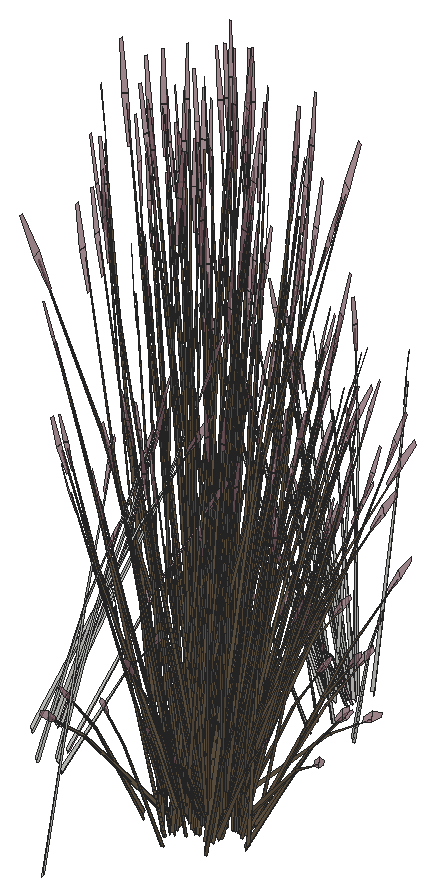
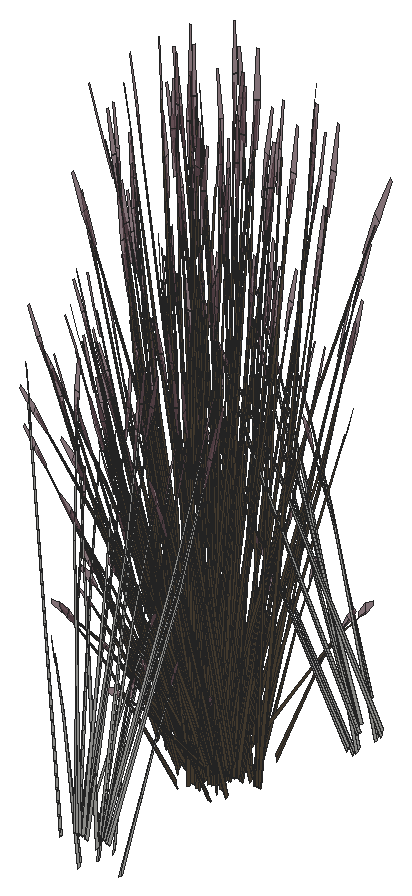
# SketchUp Ruby script. Lengths in inches.
U = 1.inch
M = Sketchup.active_model
def pt(a) = Geom::Point3d.new(a.map { |v| v * U })
def face(e, loops, mat)
  f = e.add_face(loops[0].map { |a| pt(a) })
  loops[1..].each { |l| e.add_face(l.map { |a| pt(a) }).erase! }
  f.material = f.back_material = mat if mat
  f
end
# faces: each face lists its corners as indices into pts; further lists are holes
def faces(e, pts, list, mat = nil) = list.each { |f| face(e, (f[0].is_a?(Array) ? f : [f]).map { |l| l.map { |i| pts[i] } }, mat) }
# xy, xz, yz: faces in a plane at the given z, y or x. An outline is a flat list of corners, or four numbers for a rectangle; further outlines are holes
def ring(l) = l.size == 4 ? [[l[0], l[1]], [l[2], l[1]], [l[2], l[3]], [l[0], l[3]]] : l.each_slice(2).to_a
def flat(e, list, mat, &to3) = list.each { |f| face(e, (f[0].is_a?(Array) ? f : [f]).map { |l| ring(l).map { |u, v| to3.(u, v) } }, mat) }
def xy(e, z, list, mat = nil) = flat(e, list, mat) { |x, y| [x, y, z] }
def xz(e, y, list, mat = nil) = flat(e, list, mat) { |x, z| [x, y, z] }
def yz(e, x, list, mat = nil) = flat(e, list, mat) { |y, z| [x, y, z] }
def lines(e, pts, list) = list.each { |a, b| e.add_line(pt(pts[a]), pt(pts[b])) }
# prism: a flat outline (further loops are holes) pulled along v
def prism(e, loops, v, mat = nil)
  f = face(e, loops, mat); d = Geom::Vector3d.new(v.map { |x| x * U })
  f.pushpull(f.normal.samedirection?(d) ? d.length : -d.length)
end
def box(e, o, s, mat = nil) = prism(e, [[o, [o[0] + s[0], o[1], o[2]], [o[0] + s[0], o[1] + s[1], o[2]], [o[0], o[1] + s[1], o[2]]]], [0, 0, s[2]], mat)
def at(x, y, z, deg = 0) = Geom::Transformation.translation(pt([x, y, z])) * Geom::Transformation.rotation(ORIGIN, Z_AXIS, deg.degrees)
def axes(o, x, y, z) = Geom::Transformation.new([*x, 0, *y, 0, *z, 0, *pt(o).to_a, 1])
def part(name) = M.definitions.add(name)
# library, detail: a bought-in or finely detailed component or shape, given as its bounding box
def library(name, o, s) = part(name).tap { |d| box(d.entities, o, s) }
def detail(e, o, s) = box(e.add_group.entities, o, s)
def put(e, d, t, mat = nil) = e.add_instance(d, t).tap { |i| i.material = mat if mat }
def group(e, t, mat = nil) = e.add_group.tap { |g| g.transformation = t; g.material = mat if mat }.entities
root = M.entities
M.materials.add("Forest_Floor_01_1K").color = [106, 91, 72]
M.materials.add("LightPink_Translucent").color = [144, 107, 117]
M.materials["LightPink_Translucent"].alpha = 0.75
c1 = part("blade")
p = [[2.15,0.21,22],[0,0.17,0],[0.09,0.45,0],[2.18,0.31,22],[2.29,0.31,22],[0.38,0.45,0],
  [2.48,0.24,33],[2.49,0.24,33],[2.48,0.22,33]]
faces(c1.entities,p,[[0,1,2,3],[4,5,2,3],[6,3,4,7],[8,0,3,6]])
c2 = part("seeds")
p = [[0.3,-0.1,1.38],[-0.01,-0.03,1.59],[-0.01,-0.03,0.03],[0.14,-0.07,-0.07],[0.29,-0.03,3],[0.15,0.01,3.11]]
faces(c2.entities,p,[[0,1,2,3],[1,0,4,5]],"LightPink_Translucent")
c3 = part("blade with seeds")
put(c3.entities,c1,at(0,0,0))
put(c3.entities,c2,axes([2.4,0.25,30.99],[1.5799,-0.05474,1.17369],[-0.12525,1.92788,0.29478],[-0.07173,-0.02425,1.56792]))
put(root,c3,axes([508.54,142.77,4.23],[-0.74352,0.28449,-0.1216],[-0.36538,-0.50492,-0.67495],[-0.0981,-0.21277,1.02557]))
put(root,c3,axes([507.23,125.56,1.52],[-0.70674,0.51372,0.30756],[-0.70717,-0.50832,-0.36492],[-0.02468,-0.14589,1.64885]),"Forest_Floor_01_1K")
put(root,c3,axes([507.9,142.8,3.875],[-0.7469,-0.15318,-0.51099],[0.25601,-0.52518,-0.3958],[-0.06849,-0.21144,0.97773]))
put(root,c3,axes([500.09,120.04,5.39],[-0.27143,-0.0181,1.43002],[-0.27808,-0.48551,-0.30754],[0.33346,-0.13735,0.61141]))
put(root,c3,axes([510.14,126.98,2.52],[0.65659,0.2464,1.51261],[-0.64324,0.53082,0.59816],[-0.28812,-0.31461,1.26806]),"Forest_Floor_01_1K")
put(root,c3,axes([500.28,121.75,7.33],[0.63144,0.17046,-0.35414],[-0.18417,0.49731,0.4572],[0.25423,-0.0456,0.87481]))
put(root,c3,axes([507.64,122.51,1.96],[0.39634,0.21267,1.1486],[-0.57721,0.12784,0.84392],[-0.1235,-0.16344,0.25299]),"Forest_Floor_01_1K")
put(root,c3,axes([510.43,126.81,1.66],[-0.74193,-0.49181,-0.25192],[0.6243,-0.55226,0.5513],[-0.19979,0.05753,1.68216]),"Forest_Floor_01_1K")
put(root,c3,axes([509.08,126.33,1.4],[-0.45644,-0.51287,-0.44739],[0.69137,-0.36116,0.21531],[-0.14771,-0.06346,1.43643]),"Forest_Floor_01_1K")
put(root,c3,axes([499.06,122.82,7.78],[0.75952,0.01471,-0.71045],[-0.05101,0.61953,0.08574],[0.32177,0.06538,1.00501]))
put(root,c3,axes([507.79,127.6875,4.53],[-0.01977,0.56521,-0.7886],[-0.83252,-0.03796,0.09517],[-0.08786,0.23945,1.11556]),"Forest_Floor_01_1K")
put(root,c3,axes([500.6,121.65,4.78],[-0.48937,0.07333,1.41583],[-0.07789,-0.58369,0.08104],[0.34275,-0.08835,0.80566]))
put(root,c3,axes([507.77,129.28,1.96],[-0.01966,-0.36332,1.1486],[0.49135,0.25914,0.84392],[-0.09663,0.17317,0.25299]),"Forest_Floor_01_1K")
put(root,c3,axes([508.46,123.07,4.29],[0.84639,-0.15705,0.53763],[0.14689,0.61608,0.4433],[-0.19906,-0.18157,1.11249]),"Forest_Floor_01_1K")
put(root,c3,axes([501.13,121.27,4.29],[-0.03971,-0.09277,1.76342],[0.27541,-0.54264,-0.26939],[0.27782,-0.00781,0.30037]))
put(root,c3,axes([510.05,126.7,1.4],[-0.82508,0.03772,-0.44739],[-0.07462,-0.62614,0.21531],[-0.14771,0.06346,1.43643]),"Forest_Floor_01_1K")
put(root,c3,axes([508.17,142.9,4.17],[-0.36264,-0.49684,-0.71045],[0.74649,-0.27689,0.08574],[-0.0848,-0.24006,1.00501]))
put(root,c3,axes([498.56,121.14,6.68],[-0.31515,0.01384,1.71376],[0.20907,-0.5998,0.13857],[0.44912,0.0371,0.73262]))
put(root,c3,axes([508.66,123.2,3.92],[0.34533,-0.38816,0.0643],[0.49176,0.22599,0.50621],[-0.15898,-0.12445,0.77189]),"Forest_Floor_01_1K")
put(root,c3,axes([507.4,110.87,2.56],[0.01669,-0.31544,1.54345],[0.75083,0.16661,0.21329],[-0.06506,0.33618,0.72882]))
put(root,c3,axes([508.48,127.75,1.67],[0.7111,0.30552,0.49651],[-0.42504,0.54784,0],[-0.16196,-0.06958,1.57504]),"Forest_Floor_01_1K")
put(root,c3,axes([507.51,128.49,2.56],[0.01669,-0.31544,1.54345],[0.75083,0.16661,0.21329],[-0.06506,0.33618,0.72882]),"Forest_Floor_01_1K")
put(root,c3,axes([499.71,121.7,7.78],[0.66765,-0.26986,-0.71045],[0.37208,0.55551,0.08574],[0.32259,-0.0631,1.00501]))
put(root,c3,axes([509.15,126.63,1.63],[0.20138,-0.72405,-0.23429],[0.95485,0.12621,0.51271],[-0.16685,-0.09999,1.5644]),"Forest_Floor_01_1K")
put(root,c3,axes([508.32,142.97,4.24],[-0.22906,0.4699,0.35414],[-0.66828,-0.13705,-0.4572],[-0.06128,-0.18919,0.87481]))
put(root,c3,axes([509.5,126.8,1.81],[-0.14658,0.54532,0.1448],[-0.71613,-0.09466,-0.41347],[-0.13033,-0.05599,1.26744]),"Forest_Floor_01_1K")
put(root,c3,axes([509.41,122.05,3.91],[-0.11621,-0.08567,1.74944],[-0.77555,0.05431,-0.27667],[-0.12378,-0.20491,0.14031]),"Forest_Floor_01_1K")
put(root,c3,axes([510.92,128.32,1.21],[-0.7111,0.30552,-0.49651],[-0.42504,-0.54784,0],[-0.16196,0.06958,1.57504]),"Forest_Floor_01_1K")
put(root,c3,axes([506.71,125.27,1.21],[0,-0.61104,-0.49651],[0.85008,0,0],[0,-0.13917,1.57504]),"Forest_Floor_01_1K")
put(root,c3,axes([507.08,125.84,1.67],[0,0.61104,0.49651],[-0.85008,0,0],[0,-0.13917,1.57504]),"Forest_Floor_01_1K")
put(root,c3,axes([510.97,128.16,1.39],[-0.46912,-0.61443,-0.05142],[0.79476,-0.34146,0.51607],[-0.19584,0.0585,1.6363]),"Forest_Floor_01_1K")
put(root,c3,axes([507.96,127.875,4.2],[0.54391,0.41056,-0.5672],[-0.57458,0.35956,-0.43934],[-0.08276,0.2086,1.08528]),"Forest_Floor_01_1K")
put(root,c3,axes([510.75,128.08,1.22],[-0.70886,-0.15119,-0.30978],[0.17848,-0.53243,0.30978],[-0.1429,0.0614,1.38974]),"Forest_Floor_01_1K")
put(root,c3,axes([507.72,127.57,4.24],[0.5141,-0.32171,0.35414],[0.48666,0.36734,-0.4572],[-0.07405,0.18664,0.87481]),"Forest_Floor_01_1K")
put(root,c3,axes([500.74,122.52,5.39],[-0.18299,-0.15028,1.43002],[0.23809,-0.49714,-0.30754],[0.37023,0.06735,0.61141]))
put(root,c3,axes([508.93,125.98,1.86],[-0.85568,-0.29155,-0.29095],[0.41201,-0.61537,-0.50002],[-0.02689,-0.15109,1.59708]),"Forest_Floor_01_1K")
put(root,c3,axes([511.16,125.8,2.03],[-0.02076,-0.57531,1.41272],[0.93937,0.14913,0.59816],[-0.22217,0.31481,1.3335]),"Forest_Floor_01_1K")
put(root,c3,axes([507.55,141.8,0.6875],[-0.12744,0.02202,1.76342],[-0.70477,-0.24781,-0.26939],[0.01183,-0.2067,0.30037]))
put(root,c3,axes([507.39,127.66,4.59],[0.83505,0.03027,-0.13498],[-0.02282,0.57322,-0.74919],[-0.05801,0.22077,1.13838]),"Forest_Floor_01_1K")
put(root,c3,axes([508.24,142.48,3.72],[0.22906,-0.4699,-0.35414],[0.66828,0.13705,0.4572],[-0.06128,-0.18919,0.87481]))
put(root,c3,axes([507.37,128.49,2.02],[0.69024,-0.1082,0.06507],[0.15868,0.43593,-0.86304],[-0.04376,0.22067,0.7736]),"Forest_Floor_01_1K")
put(root,c3,axes([510.63,126.53,1.86],[0.08854,0.69723,-0.29095],[-0.92215,0.04216,-0.50002],[-0.16238,0.09287,1.59708]),"Forest_Floor_01_1K")
put(root,c3,axes([508.55,125.36,1.29],[-0.31203,-0.62659,-0.69835],[0.89884,-0.22566,-0.18329],[-0.03449,-0.21218,1.54149]),"Forest_Floor_01_1K")
put(root,c3,axes([510.59,123.37,4.23],[-0.74352,0.28449,-0.1216],[-0.36538,-0.50492,-0.67495],[-0.0981,-0.21277,1.02557]),"Forest_Floor_01_1K")
put(root,c3,axes([509.96,123.4,3.875],[-0.7469,-0.15318,-0.51099],[0.25601,-0.52518,-0.3958],[-0.06849,-0.21144,0.97773]),"Forest_Floor_01_1K")
put(root,c3,axes([508.58,127.29,3.07],[-0.0186,-0.23452,1.71376],[0.80601,0.15558,0.13857],[-0.04985,0.33422,0.73262]),"Forest_Floor_01_1K")
put(root,c3,axes([507.08,125.29,1.22],[0.53038,-0.38124,-0.30978],[0.53038,0.38124,0.30978],[0,-0.1228,1.38974]),"Forest_Floor_01_1K")
put(root,c3,axes([509.47,122.82,1.32],[-0.52505,0.35054,-0.03893],[-0.48109,-0.38392,-0.17649],[-0.03387,-0.10878,0.58215]),"Forest_Floor_01_1K")
put(root,c3,axes([509.26,126.28,1.55],[0.96033,0.12874,0.45755],[-0.19544,0.7271,0.17955],[-0.14034,-0.07021,1.58856]),"Forest_Floor_01_1K")
put(root,c3,axes([509.01,126.15,1.91],[-0.36864,0.55059,0.44739],[-0.76598,-0.26498,-0.21531],[0,-0.12692,1.43643]),"Forest_Floor_01_1K")
put(root,c3,axes([510.23,123.5,4.17],[-0.36264,-0.49684,-0.71045],[0.74649,-0.27689,0.08574],[-0.0848,-0.24006,1.00501]),"Forest_Floor_01_1K")
put(root,c3,axes([508.52,142.54,3.92],[0.55987,-0.20767,0.0643],[0.27403,0.37869,0.50621],[-0.05407,-0.16693,0.77189]))
put(root,c3,axes([508.33,142.58,3.93],[0.74868,0.15974,0.48003],[-0.25601,0.52518,0.3958],[-0.04499,-0.20653,0.9933]))
put(root,c3,axes([508.74,127.44,1.67],[0.81646,-0.16218,0.17642],[0.20161,0.60355,0.35086],[-0.07282,-0.08794,1.60407]),"Forest_Floor_01_1K")
put(root,c3,axes([509.79,127.54,1.39],[-0.76598,-0.27433,0],[0.36864,-0.57001,0],[0,0,1.62707]),"Forest_Floor_01_1K")
put(root,c3,axes([510.37,123.57,4.24],[-0.22906,0.4699,0.35414],[-0.66828,-0.13705,-0.4572],[-0.06128,-0.18919,0.87481]),"Forest_Floor_01_1K")
put(root,c3,axes([511.57,128.22,1.57],[0.47504,0.61229,0],[-0.79476,0.34146,-0.51607],[-0.18101,0.07777,1.63711]),"Forest_Floor_01_1K")
put(root,c3,axes([509.15,128.49,4.26],[-0.74868,-0.15974,0.53283],[0.25601,-0.52518,0.43934],[0.04499,0.20653,1.10256]),"Forest_Floor_01_1K")
put(root,c3,axes([508.95,128.53,3.92],[-0.55987,0.20767,0.0643],[-0.27403,-0.37869,0.50621],[0.05407,0.16693,0.77189]),"Forest_Floor_01_1K")
put(root,c3,axes([511.17,127.47,1.67],[0.21949,-0.60727,0.17642],[0.8032,0.17185,0.35086],[-0.13875,0.00296,1.60407]),"Forest_Floor_01_1K")
put(root,c3,axes([510.8,126.67,1.81],[0.56134,0.36712,0.1448],[-0.46823,0.41419,-0.41347],[-0.13033,0.05599,1.26744]),"Forest_Floor_01_1K")
put(root,c3,axes([510.6,126.22,1.49],[-0.70674,-0.52593,-0.06131],[0.70717,-0.52625,0],[-0.02468,-0.01837,1.75571]),"Forest_Floor_01_1K")
put(root,c3,axes([510.79,126.4,1.91],[0.82508,-0.03772,0.44739],[0.07462,0.62614,-0.21531],[-0.14771,0.06346,1.43643]),"Forest_Floor_01_1K")
put(root,c3,axes([508.36,141.48,1.96],[0.09747,0.35631,1.1486],[-0.54071,-0.19735,0.84392],[0.05818,-0.18244,0.25299]))
put(root,c3,axes([510.99,127.84,1.52],[0.95122,0.19861,0.30756],[-0.23797,0.7099,-0.36492],[-0.15744,0.08885,1.64885]),"Forest_Floor_01_1K")
put(root,c3,axes([509.6,122.39,0.6875],[-0.12744,0.02202,1.76342],[-0.70477,-0.24781,-0.26939],[0.01183,-0.2067,0.30037]),"Forest_Floor_01_1K")
put(root,c3,axes([511.4,127.8,1.67],[0.7111,-0.30552,0.49651],[0.42504,0.54784,0],[-0.16196,0.06958,1.57504]),"Forest_Floor_01_1K")
put(root,c3,axes([510.3,123.07,3.72],[0.22906,-0.4699,-0.35414],[0.66828,0.13705,0.4572],[-0.06128,-0.18919,0.87481]),"Forest_Floor_01_1K")
put(root,c3,axes([509.18,125.61,1.55],[0.33034,0.68327,0.45755],[-0.94388,0.2376,0.17955],[0.01154,-0.12555,1.58856]),"Forest_Floor_01_1K")
put(root,c3,axes([509.02,125.52,1.4],[0.36864,-0.55059,-0.44739],[0.76598,0.26498,0.21531],[0,-0.12692,1.43643]),"Forest_Floor_01_1K")
put(root,c3,axes([509.97,127.3,1.4],[-0.24791,-0.5268,0],[0.70791,-0.18448,0],[0,0,1.54371]),"Forest_Floor_01_1K")
put(root,c3,axes([509.07,128.41,0.6875],[0.12297,-0.03325,1.76342],[0.73967,0.18301,-0.26939],[0.02163,0.20626,0.30037]),"Forest_Floor_01_1K")
put(root,c3,axes([509.23,128.6,3.72],[-0.22906,0.4699,-0.35414],[-0.66828,-0.13705,0.4572],[0.06128,0.18919,0.87481]),"Forest_Floor_01_1K")
put(root,c3,axes([510.68,142.0625,3.9],[-0.07716,0.04667,1.77383],[-0.75601,-0.15746,-0.16761],[-0.02737,-0.20368,0.31391]))
put(root,c3,axes([510.09,143.41,4.23],[-0.83505,-0.03027,-0.1216],[0.02282,-0.57322,-0.67495],[0.05801,-0.22077,1.02557]))
put(root,c3,axes([509.76,143.5,4.24],[-0.5141,0.32171,0.35414],[-0.48666,-0.36734,-0.4572],[0.07405,-0.18664,0.87481]))
put(root,c3,axes([510.97,126.26,1.4],[-0.36864,0.55059,-0.44739],[-0.76598,-0.26498,0.21531],[0,0.12692,1.43643]),"Forest_Floor_01_1K")
put(root,c3,axes([509.52,143.2,3.875],[-0.54391,-0.41056,-0.51099],[0.57458,-0.35956,-0.3958],[0.08276,-0.2086,0.97773]))
put(root,c3,axes([510.58,123.14,3.92],[0.55987,-0.20767,0.0643],[0.27403,0.37869,0.50621],[-0.05407,-0.16693,0.77189]),"Forest_Floor_01_1K")
put(root,c3,axes([508.76,129.43,3.91],[0.09631,0.0984,1.74944],[0.77725,0.03866,-0.27667],[0.07816,0.217,0.14031]),"Forest_Floor_01_1K")
put(root,c3,axes([512.43,125.93,1.67],[-0.59697,-0.44509,0.17642],[0.60159,-0.4317,0.35086],[-0.06593,0.0909,1.60407]),"Forest_Floor_01_1K")
put(root,c3,axes([510.36,125.67,1.4],[0,-0.70701,0],[0.95008,0,0],[0,0,1.79456]),"Forest_Floor_01_1K")
put(root,c3,axes([510.38,123.18,3.93],[0.74868,0.15974,0.48003],[-0.25601,0.52518,0.3958],[-0.04499,-0.20653,0.9933]),"Forest_Floor_01_1K")
put(root,c3,axes([509.48,125.8,1.625],[0.8561,0.29616,0.24065],[-0.41201,0.61537,0.50002],[0,-0.14185,1.60543]),"Forest_Floor_01_1K")
put(root,c3,axes([510.84,125.95,1.48],[0,0.70667,-0.05637],[-0.95008,0,0],[0,0.02221,1.79368]),"Forest_Floor_01_1K")
put(root,c3,axes([509.21,125.38,1.91],[-0.82508,0.03772,0.44739],[-0.07462,-0.62614,-0.21531],[0.14771,-0.06346,1.43643]),"Forest_Floor_01_1K")
put(root,c3,axes([509.16,128.1,4.24],[0.22906,-0.4699,0.35414],[0.66828,0.13705,-0.4572],[0.06128,0.18919,0.87481]),"Forest_Floor_01_1K")
put(root,c3,axes([508.82,124.31,1.67],[-0.21949,0.60727,0.17642],[-0.8032,-0.17185,0.35086],[0.13875,-0.00296,1.60407]),"Forest_Floor_01_1K")
put(root,c3,axes([510.39,127.32,1.48],[0.33034,0.70197,-0.06012],[-0.94388,0.24598,0],[0.01154,0.02451,1.72173]),"Forest_Floor_01_1K")
put(root,c3,axes([509.16,142.47,1.78],[-0.21597,0.12368,1.43002],[-0.64681,-0.21647,-0.30754],[0.1199,-0.26922,0.61141]))
put(root,c3,axes([508.43,123.56,1.57],[-0.47504,-0.61229,0],[0.79476,-0.34146,-0.51607],[0.18101,-0.07777,1.63711]),"Forest_Floor_01_1K")
put(root,c3,axes([509.3,128.17,4.17],[0.36264,0.49684,-0.71045],[-0.74649,0.27689,0.08574],[0.0848,0.24006,1.00501]),"Forest_Floor_01_1K")
put(root,c3,axes([513.12,126.4,1.39],[-0.94962,-0.00489,-0.04976],[0,-0.68292,0.49943],[-0.02984,0.15546,1.58352]),"Forest_Floor_01_1K")
put(root,c3,axes([511.25,124.34,1.67],[-0.81646,0.16218,0.17642],[-0.20161,-0.60355,0.35086],[0.07282,0.08794,1.60407]),"Forest_Floor_01_1K")
put(root,c3,axes([509.68,143.38,4.17],[0.01977,-0.56521,-0.71045],[0.83252,0.03796,0.08574],[0.08786,-0.23945,1.00501]))
put(root,c3,axes([510.42,122.08,1.96],[0.09747,0.35631,1.1486],[-0.54071,-0.19735,0.84392],[0.05818,-0.18244,0.25299]),"Forest_Floor_01_1K")
put(root,c3,axes([510.06,129.78,4.84],[0.52505,-0.35054,-0.06488],[0.48109,0.38392,-0.29416],[0.03387,0.10878,0.97024]),"Forest_Floor_01_1K")
put(root,c3,axes([509.91,125.22,1.55],[-0.62999,0.55453,0.45755],[-0.74845,-0.4895,0.17955],[0.15188,-0.05534,1.58856]),"Forest_Floor_01_1K")
put(root,c3,axes([510.99,126.1,1.41],[0.53038,0.39469,0],[-0.53038,0.39469,0],[0,0,1.69266]),"Forest_Floor_01_1K")
put(root,c3,axes([510.98,125.64,1.91],[0.36864,-0.55059,0.44739],[0.76598,0.26498,-0.21531],[0,0.12692,1.43643]),"Forest_Floor_01_1K")
put(root,c3,axes([510.66,127.55,1.4],[0.76598,0.27433,0],[-0.36864,0.57001,0],[0,0,1.74954]),"Forest_Floor_01_1K")
put(root,c3,axes([509.57,128.27,3.875],[0.7469,0.15318,-0.51099],[-0.25601,0.52518,-0.3958],[0.06849,0.21144,0.97773]),"Forest_Floor_01_1K")
put(root,c3,axes([508.93,128.3,4.23],[0.74352,-0.28449,-0.1216],[0.36538,0.50492,-0.67495],[0.0981,0.21277,1.02557]),"Forest_Floor_01_1K")
put(root,c3,axes([510.73,125.5,1.57],[-0.96033,-0.12874,0.49198],[0.19544,-0.7271,0.19306],[0.14034,0.07021,1.70813]),"Forest_Floor_01_1K")
put(root,c3,axes([512.73,122.66,3.9],[-0.07716,0.04667,1.77383],[-0.75601,-0.15746,-0.16761],[-0.02737,-0.20368,0.31391]),"Forest_Floor_01_1K")
put(root,c3,axes([512.14,124.01,4.23],[-0.83505,-0.03027,-0.1216],[0.02282,-0.57322,-0.67495],[0.05801,-0.22077,1.02557]),"Forest_Floor_01_1K")
put(root,c3,axes([512.92,126.5,1.22],[-0.53038,0.38124,-0.30978],[-0.53038,-0.38124,0.30978],[0,0.1228,1.38974]),"Forest_Floor_01_1K")
put(root,c3,axes([511.4,126.43,1.29],[0.2786,0.55945,-0.69212],[-0.80253,0.20149,-0.18165],[0.03079,0.18945,1.52773]),"Forest_Floor_01_1K")
put(root,c3,axes([510.03,143.04,3.72],[0.5141,-0.32171,-0.35414],[0.48666,0.36734,0.4572],[0.07405,-0.18664,0.87481]))
put(root,c3,axes([511.01,125.83,1.4],[0.85008,0,0],[0,0.63259,0],[0,0,1.78407]),"Forest_Floor_01_1K")
put(root,c3,axes([510.22,143.21,3.92],[0.62439,0.02847,0.0643],[-0.01712,0.42991,0.50621],[0.06534,-0.16468,0.77189]))
put(root,c3,axes([511.8125,124.1,4.24],[-0.5141,0.32171,0.35414],[-0.48666,-0.36734,-0.4572],[0.07405,-0.18664,0.87481]),"Forest_Floor_01_1K")
put(root,c3,axes([510.19,125.13,1.91],[-0.45644,-0.51287,0.44739],[0.69137,-0.36116,-0.21531],[0.14771,0.06346,1.43643]),"Forest_Floor_01_1K")
put(root,c3,axes([509.36,125.25,1.86],[-0.08854,-0.69723,-0.29095],[0.92215,-0.04216,-0.50002],[0.16238,-0.09287,1.59708]),"Forest_Floor_01_1K")
put(root,c3,axes([511.3,125.76,1.81],[0.70791,-0.1782,0.1448],[0.24791,0.50885,-0.41347],[0,0.11199,1.26744]),"Forest_Floor_01_1K")
put(root,c3,axes([511.57,123.79,3.875],[-0.54391,-0.41056,-0.51099],[0.57458,-0.35956,-0.3958],[0.08276,-0.2086,0.97773]),"Forest_Floor_01_1K")
put(root,c3,axes([510.84,142.5,3.91],[-0.00733,-0.12161,1.74944],[-0.61946,-0.35147,-0.27667],[0.09577,-0.21306,0.14031]))
put(root,c3,axes([510.03,143.17,3.93],[0.54105,0.41691,0.48003],[-0.57458,0.35956,0.3958],[0.0998,-0.1956,0.9933]))
put(root,c3,axes([511.0625,125.8,1.86],[0.85568,0.29155,-0.29095],[-0.41201,0.61537,-0.50002],[0.02689,0.15109,1.59708]),"Forest_Floor_01_1K")
put(root,c3,axes([509.24,123.71,1.22],[0.70886,0.15119,-0.30978],[-0.17848,0.53243,0.30978],[0.1429,-0.0614,1.38974]),"Forest_Floor_01_1K")
put(root,c3,axes([511.21,123.07,1.78],[-0.21597,0.12368,1.43002],[-0.64681,-0.21647,-0.30754],[0.1199,-0.26922,0.61141]),"Forest_Floor_01_1K")
put(root,c3,axes([512.92,125.94,1.67],[0,-0.61104,0.49651],[0.85008,0,0],[0,0.13917,1.57504]),"Forest_Floor_01_1K")
put(root,c3,axes([513.28,126.51,1.21],[0,0.61104,-0.49651],[-0.85008,0,0],[0,0.13917,1.57504]),"Forest_Floor_01_1K")
put(root,c3,axes([511.01,128.36,3.93],[-0.75571,0.14023,0.48003],[-0.13115,-0.55007,0.3958],[0.17773,0.16212,0.9933]),"Forest_Floor_01_1K")
put(root,c3,axes([509.07,123.47,1.21],[0.7111,-0.30552,-0.49651],[0.42504,0.54784,0],[0.16196,-0.06958,1.57504]),"Forest_Floor_01_1K")
put(root,c3,axes([510.87,128.47,3.92],[-0.34533,0.38816,0.0643],[-0.49176,-0.22599,0.50621],[0.15898,0.12445,0.77189]),"Forest_Floor_01_1K")
put(root,c3,axes([510,127.19,3.07],[-0.17368,-0.19618,1.71376],[0.80256,-0.16516,0.13857],[0.18139,0.30799,0.73262]),"Forest_Floor_01_1K")
put(root,c3,axes([510.5,124.98,1.81],[0.14658,-0.54532,0.1448],[0.71613,0.09466,-0.41347],[0.13033,0.05599,1.26744]),"Forest_Floor_01_1K")
put(root,c3,axes([508.75,143.1,3.07],[-0.14147,0.21002,1.71376],[-0.59349,-0.43464,0.13857],[0.26773,-0.27089,0.73262]))
put(root,c3,axes([511.52,124.03,1.67],[-0.7111,-0.30552,0.49651],[0.42504,-0.54784,0],[0.16196,0.06958,1.57504]),"Forest_Floor_01_1K")
put(root,c3,axes([511.74,123.98,4.17],[0.01977,-0.56521,-0.71045],[0.83252,0.03796,0.08574],[0.08786,-0.23945,1.00501]),"Forest_Floor_01_1K")
put(root,c3,axes([510.9,127.23,1.38],[0.79769,-0.20732,-0.19198],[0.2803,0.59721,0.00008],[0.08805,-0.02292,1.73897]),"Forest_Floor_01_1K")
put(root,c3,axes([510.76,128.02,4.24],[-0.11735,-0.49217,0.35414],[0.67083,-0.12996,-0.4572],[0.18018,0.14104,0.87481]),"Forest_Floor_01_1K")
put(root,c3,axes([510.67,142.85,0.6875],[-0.11372,-0.04814,1.76342],[-0.29211,-0.53779,-0.26939],[0.19706,-0.14594,0.30037]))
put(root,c3,axes([510.91,125.45,1.4],[0.45644,0.51287,-0.44739],[-0.69137,0.36116,0.21531],[0.14771,0.06346,1.43643]),"Forest_Floor_01_1K")
put(root,c3,axes([511.21,125.19,3.67],[-0.65655,-0.31748,1.38283],[0.69326,-0.49431,0.59665],[0.21183,0.29789,1.33663]),"Forest_Floor_01_1K")
put(root,c3,axes([512.08,123.64,3.72],[0.5141,-0.32171,-0.35414],[0.48666,0.36734,0.4572],[0.07405,-0.18664,0.87481]),"Forest_Floor_01_1K")
put(root,c3,axes([510.11,128.71,3.9],[0.00225,-0.07398,1.77383],[0.65113,-0.32638,-0.16761],[0.22617,0.1165,0.31391]),"Forest_Floor_01_1K")
put(root,c3,axes([512.28,123.81,3.92],[0.62439,0.02847,0.0643],[-0.01712,0.42991,0.50621],[0.06534,-0.16468,0.77189]),"Forest_Floor_01_1K")
put(root,c3,axes([512.2,127.78,1.96],[-0.4278,-0.1757,1.1486],[0.5524,-0.17852,0.84392],[0.14899,0.15122,0.25299]),"Forest_Floor_01_1K")
put(root,c3,axes([510.68,127.59,1.78],[0.01341,-0.20255,1.43002],[0.64074,-0.22625,-0.30754],[0.1978,0.24243,0.61141]),"Forest_Floor_01_1K")
put(root,c3,axes([512.9,123.1,3.91],[-0.00733,-0.12161,1.74944],[-0.61946,-0.35147,-0.27667],[0.09577,-0.21306,0.14031]),"Forest_Floor_01_1K")
put(root,c3,axes([509.92,124.72,1.25],[0.51177,-0.45928,-0.62353],[0.63575,0.41646,-0.16365],[0.20507,-0.11457,1.37633]),"Forest_Floor_01_1K")
put(root,c3,axes([512.08,123.77,3.93],[0.54105,0.41691,0.48003],[-0.57458,0.35956,0.3958],[0.0998,-0.1956,0.9933]),"Forest_Floor_01_1K")
put(root,c3,axes([512.16,124.3125,1.22],[0.17848,0.53243,-0.30978],[-0.70886,0.15119,0.30978],[0.1429,0.0614,1.38974]),"Forest_Floor_01_1K")
put(root,c3,axes([513.5,126.05,1.57],[0.95008,0,0],[0,0.68292,-0.51607],[0,0.15554,1.63711]),"Forest_Floor_01_1K")
put(root,c3,axes([510.43,125.16,1.86],[0.76714,-0.40567,-0.29095],[0.51013,0.57321,-0.50002],[0.18927,0.05821,1.59708]),"Forest_Floor_01_1K")
put(root,c3,axes([512.27,128.58,1.86],[-0.48723,-0.01916,1.0506],[0.32177,-0.40701,0.58006],[0.19248,0.1446,0.8241]),"Forest_Floor_01_1K")
put(root,c3,axes([512.7,125.09,4.24],[-0.66138,0.08733,0.35414],[-0.17464,-0.49921,-0.4572],[0.18953,-0.13408,0.87481]),"Forest_Floor_01_1K")
put(root,c3,axes([510.8,123.7,3.07],[-0.14147,0.21002,1.71376],[-0.59349,-0.43464,0.13857],[0.26773,-0.27089,0.73262]),"Forest_Floor_01_1K")
put(root,c3,axes([510.7,128.28,4.23],[0.45276,-0.52302,-0.1216],[0.65568,0.30132,-0.67495],[0.22792,0.14777,1.02557]),"Forest_Floor_01_1K")
put(root,c3,axes([510.67,144.37,4.17],[0.39688,-0.48213,-0.71045],[0.69548,0.34264,0.08574],[0.23697,-0.17468,1.00501]))
put(root,c3,axes([508.49,124.8,0.79],[-0.74787,0.24464,1.28929],[-0.23804,-0.70192,0.50096],[0.45924,0.01168,1.46642]),"Forest_Floor_01_1K")
put(root,c3,axes([513.05,125.14,4.23],[-0.70283,-0.33692,-0.1216],[0.40491,-0.48793,-0.67495],[0.19857,-0.16961,1.02557]),"Forest_Floor_01_1K")
put(root,c3,axes([511.24,128.02,3.875],[0.74975,-0.14525,-0.51099],[0.13115,0.55007,-0.3958],[0.20138,0.15763,0.97773]),"Forest_Floor_01_1K")
put(root,c3,axes([511.93,123.71,1.57],[0.47504,-0.61229,0],[0.79476,0.34146,-0.51607],[0.18101,0.07777,1.63711]),"Forest_Floor_01_1K")
put(root,c3,axes([512.72,123.45,0.6875],[-0.11372,-0.04814,1.76342],[-0.29211,-0.53779,-0.26939],[0.19706,-0.14594,0.30037]),"Forest_Floor_01_1K")
put(root,c3,axes([512.1,127.36,4.24],[-0.43232,-0.38257,0.35414],[0.49364,-0.36215,-0.4572],[0.25081,0.0551,0.87481]),"Forest_Floor_01_1K")
put(root,c3,axes([512.36,124.08,1.21],[0.7111,0.30552,-0.49651],[-0.42504,0.54784,0],[0.16196,0.06958,1.57504]),"Forest_Floor_01_1K")
put(root,c3,axes([512.49,127.71,3.92],[-0.03826,0.46465,0.0643],[-0.57772,-0.01274,0.50621],[0.2213,0.04862,0.77189]),"Forest_Floor_01_1K")
put(root,c3,axes([512.32,128.43,0.6875],[0.05536,-0.08822,1.76342],[0.69692,-0.25981,-0.26939],[0.21129,0.13447,0.30037]),"Forest_Floor_01_1K")
put(root,c3,axes([512.54,127.56,3.93],[-0.56024,0.40262,0.48003],[-0.48318,-0.42758,0.3958],[0.26285,0.07427,0.9933]),"Forest_Floor_01_1K")
put(root,c3,axes([512.7,124.74,3.875],[-0.19519,-0.55794,-0.51099],[0.73919,-0.0976,-0.3958],[0.21183,-0.14986,0.97773]),"Forest_Floor_01_1K")
put(root,c3,axes([514,127.62,3.12],[-0.14542,-0.51365,-0.03492],[0.68734,-0.11809,-0.15832],[0.14353,0.03256,0.52218]),"Forest_Floor_01_1K")
put(root,c3,axes([512.81,126.29,4.24],[-0.63144,-0.17046,0.35414],[0.18417,-0.49731,-0.4572],[0.25423,-0.0456,0.87481]),"Forest_Floor_01_1K")
put(root,c3,axes([511.32,125.25,1.25],[0.79037,0.10018,-0.62353],[-0.16679,0.61794,-0.16365],[0.23587,0.07488,1.37633]),"Forest_Floor_01_1K")
put(root,c3,axes([514.6875,125.62,1.45],[-0.47106,-0.39072,-0.06488],[0.51591,-0.35801,-0.29416],[0.14618,-0.02521,0.97024]),"Forest_Floor_01_1K")
put(root,c3,axes([513.61,123.63,1.96],[-0.25308,0.31105,1.1486],[-0.21753,-0.4179,0.84392],[0.20902,-0.10472,0.25299]),"Forest_Floor_01_1K")
put(root,c3,axes([513.3,125.01,3.92],[0.52161,0.25698,0.0643],[-0.30368,0.36595,0.50621],[0.16723,-0.11831,0.77189]),"Forest_Floor_01_1K")
put(root,c3,axes([513.16,124.91,3.93],[0.18844,0.56237,0.48003],[-0.73919,0.0976,0.3958],[0.21785,-0.13226,0.9933]),"Forest_Floor_01_1K")
put(root,c3,axes([511.16,126.58,3.07],[-0.28223,-0.10528,1.71376],[0.58406,-0.44165,0.13857],[0.36402,0.19924,0.73262]),"Forest_Floor_01_1K")
put(root,c3,axes([514.78,124.99,3.9],[-0.09924,-0.00464,1.77383],[-0.4121,-0.49725,-0.16761],[0.1655,-0.1635,0.31391]),"Forest_Floor_01_1K")
put(root,c3,axes([513.24,124.8,3.72],[0.66138,-0.08733,-0.35414],[0.17464,0.49921,0.4572],[0.18953,-0.13408,0.87481]),"Forest_Floor_01_1K")
put(root,c3,axes([512.72,124.96,4.17],[0.39688,-0.48213,-0.71045],[0.69548,0.34264,0.08574],[0.23697,-0.17468,1.00501]),"Forest_Floor_01_1K")
put(root,c3,axes([513.38,126.44,3.92],[0.27906,0.41663,0.0643],[-0.50888,0.20393,0.50621],[0.22432,-0.04024,0.77189]),"Forest_Floor_01_1K")
put(root,c3,axes([512.71,127.56,3.72],[0.43232,0.38257,-0.35414],[-0.49364,0.36215,0.4572],[0.25081,0.0551,0.87481]),"Forest_Floor_01_1K")
put(root,c3,axes([512.22,127.6,4.23],[0.04068,-0.62141,-0.1216],[0.77029,0.01698,-0.67495],[0.29667,0.04317,1.02557]),"Forest_Floor_01_1K")
put(root,c3,axes([513.08,126.45,4.23],[-0.38229,-0.5533,-0.1216],[0.6785,-0.2719,-0.67495],[0.28593,-0.073,1.02557]),"Forest_Floor_01_1K")
put(root,c3,axes([513.33,126.29,3.93],[-0.21466,0.55714,0.48003],[-0.70573,-0.19051,0.3958],[0.27753,-0.03348,0.9933]),"Forest_Floor_01_1K")
put(root,c3,axes([512.89,127.23,3.91],[0.16299,-0.01033,1.74944],[0.44707,-0.47471,-0.27667],[0.28992,0.06266,0.14031]),"Forest_Floor_01_1K")
put(root,c3,axes([513.04,125.98,3.875],[0.20584,-0.55581,-0.51099],[0.70573,0.19051,-0.3958],[0.28414,-0.05097,0.97773]),"Forest_Floor_01_1K")
put(root,c3,axes([514.8125,126.33,1.96],[-0.46945,0.10088,1.1486],[0.22097,-0.4169,0.84392],[0.24904,0.02853,0.25299]),"Forest_Floor_01_1K")
put(root,c3,axes([513.29,124.52,1.78],[-0.27143,-0.0181,1.43002],[-0.27808,-0.48551,-0.30754],[0.33346,-0.13735,0.61141]),"Forest_Floor_01_1K")
put(root,c3,axes([513.47,126.23,3.72],[0.63144,0.17046,-0.35414],[-0.18417,0.49731,0.4572],[0.25423,-0.0456,0.87481]),"Forest_Floor_01_1K")
put(root,c3,axes([512.25,127.3,4.17],[0.75952,0.01471,-0.71045],[-0.05101,0.61953,0.08574],[0.32177,0.06538,1.00501]),"Forest_Floor_01_1K")
put(root,c3,axes([513.8,126.13,1.17],[-0.48937,0.07333,1.41583],[-0.07789,-0.58369,0.08104],[0.34275,-0.08835,0.80566]),"Forest_Floor_01_1K")
put(root,c3,axes([514.33,125.75,0.6875],[-0.03971,-0.09277,1.76342],[0.27541,-0.54264,-0.26939],[0.27782,-0.00781,0.30037]),"Forest_Floor_01_1K")
put(root,c3,axes([514.6,128.1,3.9],[-0.0687,-0.05349,1.77383],[0.15029,-0.57341,-0.16761],[0.27062,-0.03664,0.31391]),"Forest_Floor_01_1K")
put(root,c3,axes([511.75,125.62,3.07],[-0.31515,0.01384,1.71376],[0.20907,-0.5998,0.13857],[0.44912,0.0371,0.73262]),"Forest_Floor_01_1K")
put(root,c3,axes([512.91,126.18,4.17],[0.66765,-0.26986,-0.71045],[0.37208,0.55551,0.08574],[0.32259,-0.0631,1.00501]),"Forest_Floor_01_1K")
put(root,c3,axes([515.15,125.59,3.91],[0.10543,-0.09307,1.74944],[-0.13495,-0.57092,-0.27667],[0.26455,-0.10825,0.14031]),"Forest_Floor_01_1K")
put(root,c3,axes([513.93,127,1.78],[-0.18299,-0.15028,1.43002],[0.23809,-0.49714,-0.30754],[0.37023,0.06735,0.61141]),"Forest_Floor_01_1K")
